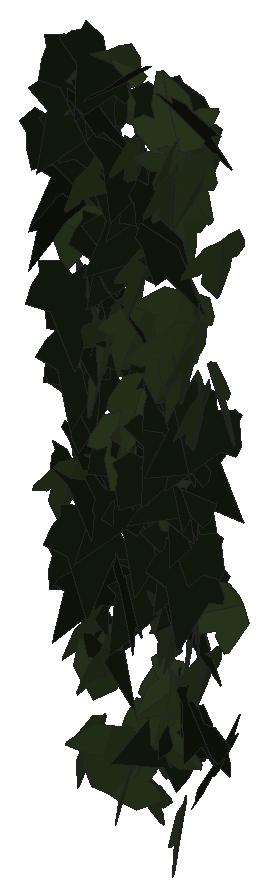
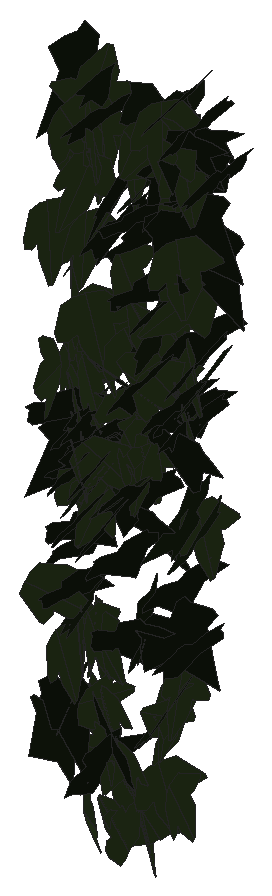
# SketchUp Ruby script. Lengths in inches.
U = 1.inch
M = Sketchup.active_model
def pt(a) = Geom::Point3d.new(a.map { |v| v * U })
def face(e, loops, mat)
  f = e.add_face(loops[0].map { |a| pt(a) })
  loops[1..].each { |l| e.add_face(l.map { |a| pt(a) }).erase! }
  f.material = f.back_material = mat if mat
  f
end
# faces: each face lists its corners as indices into pts; further lists are holes
def faces(e, pts, list, mat = nil) = list.each { |f| face(e, (f[0].is_a?(Array) ? f : [f]).map { |l| l.map { |i| pts[i] } }, mat) }
# xy, xz, yz: faces in a plane at the given z, y or x. An outline is a flat list of corners, or four numbers for a rectangle; further outlines are holes
def ring(l) = l.size == 4 ? [[l[0], l[1]], [l[2], l[1]], [l[2], l[3]], [l[0], l[3]]] : l.each_slice(2).to_a
def flat(e, list, mat, &to3) = list.each { |f| face(e, (f[0].is_a?(Array) ? f : [f]).map { |l| ring(l).map { |u, v| to3.(u, v) } }, mat) }
def xy(e, z, list, mat = nil) = flat(e, list, mat) { |x, y| [x, y, z] }
def xz(e, y, list, mat = nil) = flat(e, list, mat) { |x, z| [x, y, z] }
def yz(e, x, list, mat = nil) = flat(e, list, mat) { |y, z| [x, y, z] }
def lines(e, pts, list) = list.each { |a, b| e.add_line(pt(pts[a]), pt(pts[b])) }
# prism: a flat outline (further loops are holes) pulled along v
def prism(e, loops, v, mat = nil)
  f = face(e, loops, mat); d = Geom::Vector3d.new(v.map { |x| x * U })
  f.pushpull(f.normal.samedirection?(d) ? d.length : -d.length)
end
def box(e, o, s, mat = nil) = prism(e, [[o, [o[0] + s[0], o[1], o[2]], [o[0] + s[0], o[1] + s[1], o[2]], [o[0], o[1] + s[1], o[2]]]], [0, 0, s[2]], mat)
def at(x, y, z, deg = 0) = Geom::Transformation.translation(pt([x, y, z])) * Geom::Transformation.rotation(ORIGIN, Z_AXIS, deg.degrees)
def axes(o, x, y, z) = Geom::Transformation.new([*x, 0, *y, 0, *z, 0, *pt(o).to_a, 1])
def part(name) = M.definitions.add(name)
# library, detail: a bought-in or finely detailed component or shape, given as its bounding box
def library(name, o, s) = part(name).tap { |d| box(d.entities, o, s) }
def detail(e, o, s) = box(e.add_group.entities, o, s)
def put(e, d, t, mat = nil) = e.add_instance(d, t).tap { |i| i.material = mat if mat }
def group(e, t, mat = nil) = e.add_group.tap { |g| g.transformation = t; g.material = mat if mat }.entities
root = M.entities
M.materials.add("efeu1").color = [18, 25, 13]
M.materials.add("efeu2").color = [43, 57, 29]
c1 = part("ivyleaf_9")
p = [[1.54,2.16,1.25],[1.36,2.04,1.19],[-0.21,0.99,0.68],[-0.71,1.11,0.82],[-0.85,0.86,0.67],[-0.8,0.17,0.21],
  [-0.9,-0.01,0.1],[-0.67,-0.16,-0.02],[-0.08,-0.08,-0.05],[-0.03,-0.6,-0.4],[0.65,-0.88,-0.66],[0.83,-0.6,-0.49],
  [1.29,-0.42,-0.43],[1.8125,-0.07,-0.26],[1.21,0.44,0.15]]
faces(c1.entities,p,[[0,1,2,3,4,5,6,7,8,9,10,11,12,13,14]],"efeu1")
c2 = part("ivyleaf_10")
p = [[0,0.5,-0.03],[-0.0625,2.02,-0.43],[-0.19,2.01,-0.46],[-0.54,1.05,-0.29],[-0.52,0.625,-0.18],[-0.83,0.76,-0.28],
  [-1.16,0.64,-0.33],[-1.15,0.33,-0.24],[-0.77,-0.39,0.02],[-0.3,-0.51,0.16],[0.04,-0.48,0.23],[-0.02,2.01,-0.4375],
  [-0.06,2.01,-0.43],[0.04,-0.49,0.23],[0.67,-0.49,0.14],[1.38,0.36,-0.2],[1.375,0.51,-0.24],[0.81,0.65,-0.19],
  [0.62,0.59,-0.15],[0.6,1.09,-0.28],[0.5,1.23,-0.31]]
faces(c2.entities,p,[[0,1,2,3,4,5,6,7,8,9,10],[11,12,0,13,14,15,16,17,18,19,20]],"efeu2")
put(root,c1,axes([511.84,134.85,198.29],[0.40658,-0.68072,-0.04764],[-0.0172,0.04522,-0.79285],[0.68216,0.40686,0.00841]))
put(root,c1,axes([512.53,134.11,201.56],[-0.25115,0.66674,-0.46076],[0.16514,-0.43016,-0.71247],[-0.79345,-0.30057,-0.00244]))
put(root,c2,axes([512.75,134.66,198.61],[-0.49376,0.3392,0.53412],[-0.55294,0.09802,-0.5734],[-0.30757,-0.72074,0.17339]))
put(root,c2,axes([512.46,135.24,201.67],[-0.36469,-0.72316,0.06062],[0.01379,-0.07474,-0.80861],[0.72556,-0.36206,0.04584]))
put(root,c1,axes([512.02,134.13,203.6875],[0.36365,-0.69626,-0.36319],[-0.07081,0.36954,-0.77933],[0.78209,0.35719,0.09831]))
put(root,c1,axes([512.08,135.18,190.72],[0.15879,-0.71028,-0.24214],[0.00767,0.24903,-0.72545],[0.75039,0.14776,0.05865]))
put(root,c2,axes([512.5625,134.24,193.74],[-0.14928,-0.76224,0.08694],[-0.02214,-0.08425,-0.7767],[0.76686,-0.15081,-0.0055]))
put(root,c1,axes([512.76,134.6875,202.5],[-0.11782,0.44846,-0.6909],[0.01098,-0.69702,-0.4543],[-0.82362,-0.07344,0.09278]))
put(root,c1,axes([512.18,134.89,205.34],[0.1344,-0.8279,-0.0504],[0.00197,0.05138,-0.83868],[0.82943,0.13403,0.01016]))
put(root,c1,axes([512.32,135.61,197.69],[-0.07367,-0.77956,0.11326],[0.01294,-0.11494,-0.78268],[0.78764,-0.07103,0.02346]))
put(root,c2,axes([512.29,134.83,200.39],[-0.19325,-0.42858,-0.65534],[0.52525,0.42966,-0.43588],[0.58074,-0.53123,0.17616]))
put(root,c2,axes([512.65,134.875,197.27],[0.5342,-0.60721,-0.00793],[-0.00385,0.00718,-0.80875],[0.60725,0.53421,0.00185]))
put(root,c1,axes([512.375,134.73,196.84],[0.13779,-0.76262,-0.13542],[-0.03079,0.13205,-0.77494],[0.77394,0.14103,-0.00672]))
put(root,c2,axes([512.77,134.6,203.95],[-0.21101,-0.79134,0.03752],[-0.00743,-0.03685,-0.81898],[0.79219,-0.21113,0.00231]))
put(root,c1,axes([512.45,134.38,199.14],[-0.07657,-0.77873,-0.14922],[0.01484,0.14848,-0.78249],[0.79276,-0.078,0.00023]))
put(root,c1,axes([512.34,134.59,198.43],[0.27378,-0.76195,-0.06968],[-0.01741,0.06779,-0.80962],[0.76494,0.27426,0.00652]))
put(root,c1,axes([512.27,134.875,194.3],[0.66045,-0.52357,-0.07973],[-0.05785,0.05537,-0.84277],[0.52643,0.66294,0.00742]))
put(root,c1,axes([512.89,135.05,204.72],[-0.7274,-0.39521,-0.04714],[0.0439,0.01794,-0.82782],[0.39558,-0.72871,0.00519]))
put(root,c1,axes([512.56,134.77,197.09],[-0.16271,-0.76618,0.0221],[-0.00389,-0.02177,-0.78326],[0.76649,-0.16275,0.00072]))
put(root,c1,axes([512.71,135.03,196.26],[-0.6683,-0.22136,-0.39399],[0.3706,0.13405,-0.70395],[0.25862,-0.76412,-0.00936]))
put(root,c1,axes([512.3125,134.73,193.44],[0.22589,-0.66532,0.34],[0.15308,-0.30646,-0.70138],[0.73131,0.26966,0.04179]))
put(root,c1,axes([512.84,134.54,204.52],[-0.55449,-0.59776,0.11302],[-0.00104,-0.15199,-0.80898],[0.60835,-0.5451,0.10163]))
put(root,c2,axes([512.89,134.53,189.27],[-0.06575,-0.66927,-0.36742],[0.03399,0.36585,-0.67249],[0.76274,-0.07399,-0.0017]))
put(root,c2,axes([512.82,134.87,186.02],[0.15738,-0.66374,0.32256],[0.14268,-0.29622,-0.67916],[0.72404,0.20265,0.06372]))
put(root,c2,axes([513.05,135.15,205.35],[-0.34378,-0.751,-0.03214],[0.06504,0.00549,-0.82399],[0.74887,-0.34523,0.05681]))
put(root,c2,axes([513.28,135.01,197.73],[-0.43955,-0.40842,0.52634],[-0.23248,-0.49691,-0.57973],[0.62434,-0.47257,0.15469]))
put(root,c1,axes([512.7,134.5,203.92],[-0.05034,-0.56971,-0.63941],[0.09626,0.63269,-0.5713],[0.85097,-0.10528,0.0268]))
put(root,c1,axes([513.21,134.54,190.74],[0.01969,0.42636,-0.64028],[0.00813,-0.64057,-0.4263],[-0.76921,0.00415,-0.0209]))
put(root,c1,axes([512.92,134.62,192.01],[-0.09754,-0.81237,-0.03715],[-0.00105,0.03754,-0.81819],[0.81322,-0.09739,-0.00551]))
put(root,c1,axes([512.75,135.25,188.76],[0.41153,-0.66558,-0.0595],[-0.03251,0.04986,-0.78253],[0.66744,0.41281,-0.00143]))
put(root,c2,axes([513.1,134.4375,187.97],[0.10106,0.43423,-0.7713],[0.15011,0.75665,0.44565],[0.87231,-0.18052,0.01266]))
put(root,c1,axes([513.02,135.01,205.49],[-0.17654,-0.66441,0.46982],[0.03532,-0.48655,-0.6748],[0.81297,-0.12314,0.13134]))
put(root,c2,axes([513.32,134.46,188.47],[0.00748,-0.65222,-0.3851],[0.00876,0.38517,-0.65217],[0.75738,0.00199,0.01135]))
put(root,c1,axes([512.97,135.28,200.17],[0.01245,-0.7808,0.15686],[0.04442,-0.15596,-0.77982],[0.79516,0.02094,0.0411]))
put(root,c2,axes([512.94,135.02,204.77],[-0.5749,-0.2681,-0.53427],[0.5376,0.09222,-0.62475],[0.26137,-0.77939,0.10986]))
put(root,c2,axes([513.29,134.13,202.66],[-0.043,-0.71014,-0.39764],[0.08288,0.3923,-0.70957],[0.80966,-0.07787,0.05151]))
put(root,c1,axes([513.7,134.26,205.16],[0.00036,0.82514,0.02135],[-0.14585,0.02107,-0.81216],[-0.81243,-0.00342,0.14581]))
put(root,c2,axes([513.55,134.53,186.2],[-0.39285,-0.6209,0.19031],[-0.06609,-0.18304,-0.73362],[0.64604,-0.39629,0.04067]))
put(root,c1,axes([513.19,133.87,204.87],[0.71336,-0.37155,-0.18742],[-0.09456,0.21749,-0.79108],[0.40526,0.70477,0.14532]))
put(root,c2,axes([513.44,134.34,197.54],[0.66835,-0.50532,0.29755],[0.22257,-0.19882,-0.83757],[0.54254,0.70406,-0.02296]))
put(root,c1,axes([513.4375,135.42,197.87],[0.09212,-0.7858,-0.05674],[-0.00055,0.05706,-0.79115],[0.78784,0.09192,0.00608]))
put(root,c1,axes([513.74,135.35,200.36],[-0.40139,-0.64655,0.26374],[-0.07691,-0.26143,-0.75792],[0.69402,-0.4029,0.06854]))
put(root,c1,axes([513.24,135.01,199.16],[0.51221,-0.5797,0.21818],[0.13297,-0.1736,-0.77343],[0.60496,0.52898,-0.01472]))
put(root,c1,axes([514.05,134.67,193.48],[-0.81012,-0.05819,-0.14847],[0.14793,0.01297,-0.8122],[0.05958,-0.82351,-0.0023]))
put(root,c2,axes([513.86,134.89,185.06],[0.42164,-0.61306,-0.02625],[-0.00722,0.02689,-0.74401],[0.61358,0.4216,0.00928]))
put(root,c2,axes([513.66,134.43,197.94],[-0.19601,-0.80945,0.23875],[0.13955,0.21065,0.82873],[-0.83231,0.22594,0.08272]))
put(root,c2,axes([514.03,134.73,195.35],[-0.74767,0.22882,0.1356],[-0.12249,0.06288,-0.78153],[-0.23609,-0.75726,-0.02392]))
put(root,c1,axes([513.95,135.52,202.3125],[-0.40722,-0.65943,0.22641],[0.00362,-0.2642,-0.76297],[0.6972,-0.38379,0.1362]))
put(root,c1,axes([513.75,135.12,194.6],[-0.0341,-0.74925,-0.27158],[0.04489,0.26959,-0.74939],[0.79568,-0.04732,0.03064]))
put(root,c1,axes([514.13,135.54,190.54],[-0.55504,-0.5197,-0.00477],[0.00334,0.00341,-0.76037],[0.51971,-0.55505,-0.00021]))
put(root,c2,axes([514.01,134.67,195.24],[0.58859,0.51681,-0.1362],[-0.09897,-0.0937,-0.78326],[-0.52521,0.59683,-0.00504]))
put(root,c1,axes([514.7,135.21,197.57],[-0.65671,0.35112,0.29934],[-0.33746,-0.0104,-0.72813],[-0.31466,-0.72165,0.15615]))
put(root,c2,axes([514.31,134.83,198.38],[-0.36817,-0.65439,0.27216],[-0.06466,-0.2744,-0.74724],[0.70577,-0.3665,0.07352]))
put(root,c1,axes([513.87,134.83,202.98],[-0.08017,-0.68111,0.44747],[0.10566,-0.45453,-0.67292],[0.80807,-0.00814,0.13238]))
put(root,c2,axes([513.87,134.6,184.84],[-0.61721,-0.4492,0.47082],[0.37569,0.28387,0.76333],[-0.53133,0.72252,-0.00719]))
put(root,c1,axes([513.79,134.84,190.63],[0.24049,-0.05898,-0.8232],[0.77044,-0.29137,0.24595],[-0.2959,-0.8066,-0.02865]))
put(root,c2,axes([514.32,134.77,195.48],[0.10635,-0.70765,0.32439],[0.11547,-0.30944,-0.71289],[0.76984,0.14417,0.06212]))
put(root,c1,axes([514.42,134.8,201.27],[-0.35913,-0.55118,0.48288],[-0.18072,-0.45452,-0.65322],[0.71014,-0.39441,0.07796]))
put(root,c1,axes([514.28,135.33,192.68],[-0.17392,-0.77302,0.05514],[-0.00496,-0.0554,-0.79231],[0.77497,-0.17384,0.0073]))
put(root,c2,axes([514.51,134.48,203.85],[0.11203,-0.81799,-0.13795],[0.01688,0.14143,-0.82487],[0.82937,0.10762,0.03542]))
put(root,c1,axes([514.03,135.32,194.5],[0.14811,-0.75304,0.17605],[0.22434,-0.12971,-0.74354],[0.74009,0.19001,0.19015]))
put(root,c2,axes([514.39,134.99,186.84],[0.69613,-0.36812,0.07239],[0.06268,-0.03632,-0.78747],[0.3699,0.69894,-0.00279]))
put(root,c2,axes([514.97,135.47,195.27],[-0.52616,-0.09019,0.55147],[-0.39931,-0.46919,-0.45772],[0.3909,-0.60069,0.27472]))
put(root,c2,axes([514.1,135.3125,184.57],[-0.32311,-0.11608,0.7013],[0.69993,-0.18639,0.29163],[0.12405,0.74932,0.18118]))
put(root,c2,axes([514.65,134.61,200.38],[0.11885,-0.79103,0.21126],[0.05481,-0.20531,-0.79958],[0.81692,0.12886,0.02291]))
put(root,c2,axes([514.63,134.5,196.63],[0.38952,0.64995,-0.26409],[-0.14876,-0.21867,-0.7576],[-0.6856,0.41671,0.01435]))
put(root,c1,axes([514.42,135.22,202.01],[0.16758,-0.77335,-0.15333],[-0.03253,0.14984,-0.7913],[0.78773,0.17071,-0.00006]))
put(root,c2,axes([515.16,134.875,189.75],[0.25697,-0.07163,-0.74482],[-0.53343,0.53472,-0.23547],[0.52472,0.57867,0.12538]))
put(root,c1,axes([514.65,134.91,186.37],[-0.38869,0.47204,0.48785],[0.21673,-0.44645,0.60466],[0.64331,0.43562,0.09105]))
put(root,c1,axes([514.62,135.69,193.28],[-0.01056,-0.67299,0.37796],[0.02116,-0.3781,-0.67266],[0.77157,0.00116,0.02362]))
put(root,c1,axes([514.62,135.22,195.01],[0.30814,-0.72164,0.06926],[0.01713,-0.06799,-0.7846],[0.72475,0.30842,-0.0109]))
put(root,c1,axes([515.05,135.54,186.4375],[0.15123,-0.46828,-0.67227],[0.20915,-0.63891,0.49209],[-0.79214,-0.25809,0.00158]))
put(root,c1,axes([514.94,134.45,202.6],[0.42303,-0.53796,-0.47731],[-0.31886,0.35606,-0.68391],[0.64464,0.52915,-0.02506]))
put(root,c2,axes([515.37,135.18,199.125],[-0.58908,-0.51571,0.21154],[-0.10513,-0.19947,-0.77903],[0.54741,-0.59328,0.07803]))
put(root,c2,axes([515.18,135.15,190.17],[0.17267,-0.71806,0.19471],[0.07577,-0.18187,-0.73791],[0.74012,0.18615,0.03012]))
put(root,c2,axes([515.09,135.1,193.9],[-0.73417,0.25942,-0.19684],[0.18464,-0.06827,-0.77865],[-0.26824,-0.75703,0.00276]))
put(root,c2,axes([515.125,134.8125,188.1],[0.73181,-0.31697,0.05665],[0.0522,-0.02203,-0.7975],[0.31774,0.73366,0.00053]))
put(root,c1,axes([514.95,135.43,194.87],[0.0644,-0.73438,0.20839],[0.01466,-0.2079,-0.73719],[0.76324,0.06596,-0.00342]))
put(root,c2,axes([515.28,135.14,187.99],[-0.2206,-0.06764,0.72159],[0.09809,-0.75013,-0.04033],[0.71809,0.08168,0.22719]))
put(root,c1,axes([514.89,135.13,204.95],[0.21931,-0.75212,-0.27112],[0.08331,0.3011,-0.76791],[0.79514,0.17589,0.15523]))
put(root,c1,axes([515.14,135.13,196.32],[0.18766,-0.75026,-0.16423],[-0.04641,0.15767,-0.77335],[0.76662,0.1932,-0.00662]))
put(root,c2,axes([515.36,135.26,201.48],[-0.08517,-0.81874,-0.02947],[0.21735,0.00599,-0.79447],[0.78991,-0.08992,0.21542]))
put(root,c2,axes([514.87,134.9,186.53],[-0.1442,0.00621,-0.78452],[0.72135,-0.31259,-0.13506],[-0.30848,-0.73386,0.05089]))
put(root,c2,axes([515.5,135.01,197.25],[0.20506,-0.77516,0.02329],[-0.00274,-0.02481,-0.80178],[0.77551,0.20488,-0.00899]))
put(root,c1,axes([515.375,134.95,195.45],[-0.31374,-0.68993,0.23057],[0.03134,-0.26368,-0.74639],[0.72676,-0.28647,0.13172]))
put(root,c2,axes([515.88,134.16,197.6],[0.26155,-0.2663,-0.76266],[-0.49834,0.57774,-0.37264],[0.63579,0.56239,0.02167]))
put(root,c1,axes([515.13,135.4,194.4375],[0.25858,-0.71561,0.19912],[0.07272,-0.18544,-0.76087],[0.73922,0.26856,0.00519]))
put(root,c2,axes([515.65,134.48,190.1],[0.2761,-0.54792,-0.48432],[-0.06523,0.49717,-0.59965],[0.72838,0.25222,0.12988]))
put(root,c1,axes([515.2,134.09,194.9],[0.10819,-0.64098,-0.45302],[0.1313,0.46563,-0.62747],[0.77384,0.01061,0.1698]))
put(root,c2,axes([515.77,134.21,198.36],[-0.38758,-0.69551,0.15029],[-0.01853,-0.16121,-0.79386],[0.71132,-0.38317,0.06121]))
put(root,c1,axes([515.47,135.5625,193.25],[-0.11492,-0.66719,0.38842],[0.00674,-0.39356,-0.67401],[0.77199,-0.09588,0.06371]))
put(root,c2,axes([515.75,135.26,195.29],[0.41681,-0.66314,-0.05401],[-0.02139,0.05034,-0.7832],[0.66499,0.41727,0.00866]))
put(root,c1,axes([515.76,135.65,191.32],[-0.36637,-0.59287,0.32661],[-0.09415,-0.32314,-0.69218],[0.6703,-0.36944,0.0813]))
put(root,c1,axes([515.5,135.44,194.79],[-0.01926,-0.76026,0.19273],[0.02341,-0.19326,-0.76001],[0.78396,-0.01291,0.02743]))
put(root,c2,axes([515.82,134.38,204.14],[0.22485,-0.77012,-0.20303],[-0.0111,0.20792,-0.80095],[0.79636,0.22034,0.04617]))
put(root,c2,axes([515.93,134.62,194.09],[-0.46753,-0.60687,0.21071],[-0.06946,-0.21132,-0.76275],[0.63864,-0.46725,0.0713]))
put(root,c1,axes([515.46,133.99,201.67],[0.6,-0.53386,-0.38343],[-0.24936,0.29547,-0.80159],[0.60815,0.64786,0.04962]))
put(root,c2,axes([515.66,134.84,202.86],[-0.21993,-0.6912,-0.40577],[0.2736,0.33075,-0.71171],[0.75336,-0.32191,0.14002]))
put(root,c2,axes([515.94,134.24,204.59],[0.58722,0.59892,0.13219],[-0.09667,-0.09034,0.83874],[0.60567,-0.59509,0.00571]))
put(root,c2,axes([515.93,135.07,196.67],[0.46106,-0.66138,-0.1514],[-0.0541,0.14663,-0.80529],[0.67632,0.46259,0.03879]))
put(root,c2,axes([516.17,134.26,203.83],[-0.67735,-0.4383,0.27879],[-0.21949,-0.17374,-0.80639],[0.47081,-0.71157,0.02516]))
put(root,c2,axes([516.03,135.09,204.22],[-0.14798,-0.69496,0.40224],[-0.05754,-0.39878,-0.71016],[0.8009,-0.15706,0.02329]))
put(root,c2,axes([515.98,134.59,198.66],[-0.13218,-0.76363,0.2853],[0.02313,-0.29242,-0.77198],[0.81486,-0.11557,0.06819]))
put(root,c2,axes([515.97,134.02,203.41],[0.09347,-0.81307,-0.20921],[0.00396,0.21093,-0.81798],[0.83955,0.08953,0.02715]))
put(root,c1,axes([516.14,134.98,194.36],[-0.51186,-0.41326,0.42393],[-0.25937,-0.34723,-0.65166],[0.53219,-0.5667,0.09015]))
put(root,c2,axes([515.65,134.79,184.5],[0.37612,-0.3326,0.5645],[0.41169,-0.38638,-0.50196],[0.5097,0.55752,-0.01112]))
put(root,c1,axes([516.03,135.0625,195.47],[-0.25849,-0.45142,0.61389],[-0.1831,-0.59247,-0.51276],[0.73968,-0.30441,0.08761]))
put(root,c1,axes([515.65,134.73,190.72],[0.53866,-0.57731,-0.10779],[-0.07556,0.07693,-0.78957],[0.5824,0.54392,-0.00274]))
put(root,c1,axes([516.1,134.86,192.72],[-0.44063,-0.63039,0.10894],[-0.04916,-0.09852,-0.76895],[0.63784,-0.44307,0.01599]))
put(root,c2,axes([516.13,134.64,198.21],[0.18799,-0.79558,-0.04818],[-0.01221,0.04662,-0.81749],[0.79694,0.18839,-0.00116]))
put(root,c2,axes([516.15,134.56,190.03],[0.42944,-0.58418,-0.29455],[-0.08197,0.30151,-0.7175],[0.64908,0.42458,0.10426]))
put(root,c2,axes([516.33,134.51,199.85],[0.49786,-0.40858,-0.48347],[-0.15627,0.51671,-0.5976],[0.6134,0.46326,0.24015]))
put(root,c1,axes([515.87,134.5,195.09],[-0.09114,-0.2557,-0.77693],[0.21672,0.74625,-0.27103],[0.7887,-0.23461,-0.01531]))
put(root,c1,axes([516.32,135.31,196.1875],[-0.53398,-0.57417,0.07972],[-0.05042,-0.06197,-0.78408],[0.57748,-0.53633,0.00525]))
put(root,c1,axes([516.63,134.5,187.61],[0.32371,0.19882,-0.72635],[-0.70035,-0.21114,-0.36992],[-0.27682,0.76668,0.08649]))
put(root,c2,axes([516.36,134.97,189.16],[0.03557,-0.76413,0.08481],[0.00509,-0.08467,-0.76495],[0.7688,0.03592,0.00114]))
put(root,c2,axes([516.8125,135.21,190.77],[0.33551,0.01484,-0.73285],[-0.72871,-0.08035,-0.33524],[-0.07922,0.80199,-0.02002]))
put(root,c1,axes([516.09,134.07,205.53],[0.83028,0.05338,-0.16893],[-0.17021,0.0158,-0.83158],[-0.04914,0.84714,0.02616]))
put(root,c2,axes([516.19,134.8125,190.26],[-0.27823,0.54544,-0.51617],[0.21602,-0.46906,-0.6121],[-0.71921,-0.35189,0.01584]))
put(root,c1,axes([516.24,134.55,192.05],[-0.11812,-0.78423,0.15144],[0.01075,-0.15464,-0.79239],[0.79865,-0.11391,0.03306]))
put(root,c1,axes([516.08,134.89,187.76],[0.31516,-0.19048,-0.71429],[0.59013,-0.40285,0.36781],[-0.44524,-0.66877,-0.01811]))
put(root,c2,axes([516.53,134.68,203.68],[0.10823,-0.68902,0.4656],[0.05496,-0.46257,-0.69732],[0.82977,0.12051,-0.01454]))
put(root,c2,axes([516.58,134.36,196.99],[0.15884,-0.77836,-0.1545],[-0.01211,0.15517,-0.79418],[0.79345,0.15819,0.01881]))
put(root,c2,axes([516.73,135.03,201.2],[-0.16819,-0.79744,-0.10396],[-0.00029,0.10627,-0.81469],[0.80419,-0.16674,-0.02204]))
put(root,c2,axes([516.38,135.33,197.1875],[-0.43022,0.49222,-0.54563],[0.36526,-0.40538,-0.65371],[-0.63763,-0.56433,-0.00632]))
put(root,c1,axes([516.98,134.43,186.34],[-0.45242,0.41044,-0.53673],[-0.39164,0.36708,0.61082],[0.5506,0.59835,-0.00655]))
